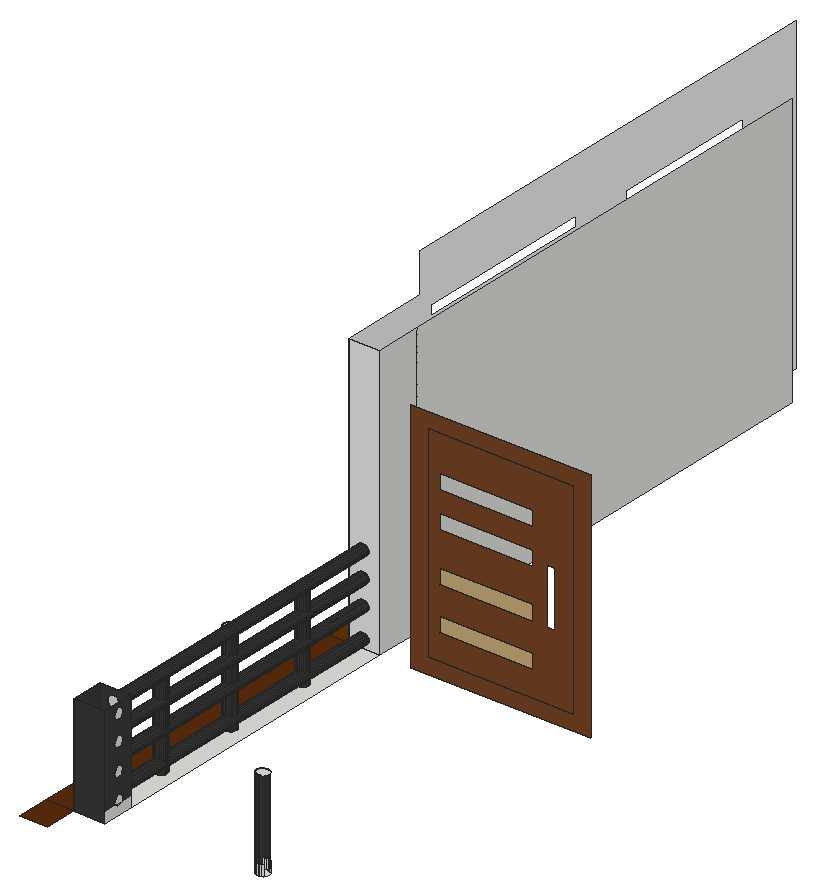
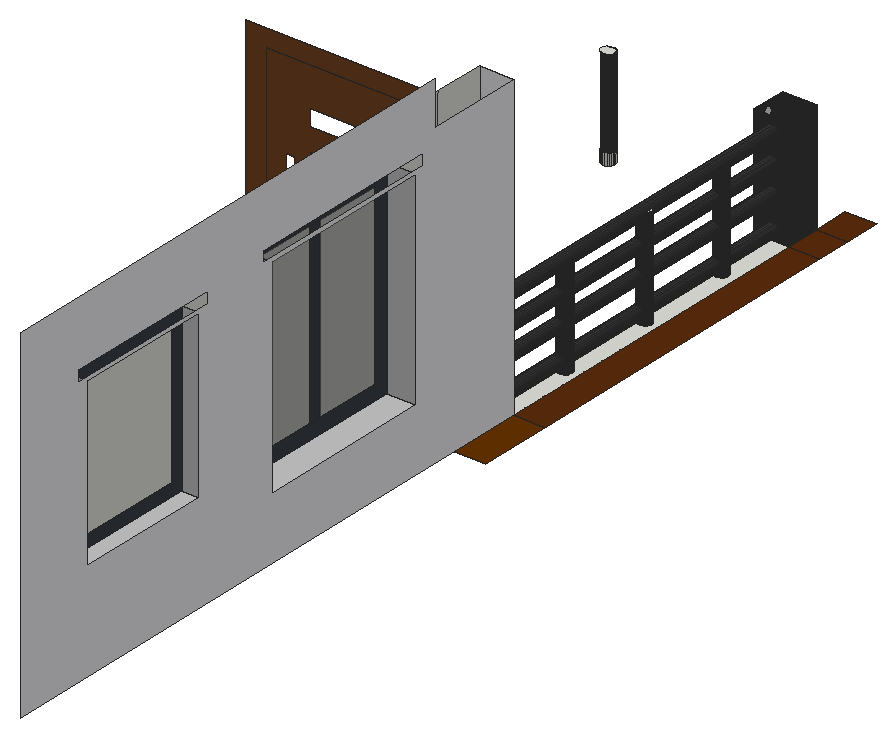
# SketchUp Ruby script. Lengths in inches.
U = 1.inch
M = Sketchup.active_model
def pt(a) = Geom::Point3d.new(a.map { |v| v * U })
def face(e, loops, mat)
  f = e.add_face(loops[0].map { |a| pt(a) })
  loops[1..].each { |l| e.add_face(l.map { |a| pt(a) }).erase! }
  f.material = f.back_material = mat if mat
  f
end
# faces: each face lists its corners as indices into pts; further lists are holes
def faces(e, pts, list, mat = nil) = list.each { |f| face(e, (f[0].is_a?(Array) ? f : [f]).map { |l| l.map { |i| pts[i] } }, mat) }
# xy, xz, yz: faces in a plane at the given z, y or x. An outline is a flat list of corners, or four numbers for a rectangle; further outlines are holes
def ring(l) = l.size == 4 ? [[l[0], l[1]], [l[2], l[1]], [l[2], l[3]], [l[0], l[3]]] : l.each_slice(2).to_a
def flat(e, list, mat, &to3) = list.each { |f| face(e, (f[0].is_a?(Array) ? f : [f]).map { |l| ring(l).map { |u, v| to3.(u, v) } }, mat) }
def xy(e, z, list, mat = nil) = flat(e, list, mat) { |x, y| [x, y, z] }
def xz(e, y, list, mat = nil) = flat(e, list, mat) { |x, z| [x, y, z] }
def yz(e, x, list, mat = nil) = flat(e, list, mat) { |y, z| [x, y, z] }
def lines(e, pts, list) = list.each { |a, b| e.add_line(pt(pts[a]), pt(pts[b])) }
# prism: a flat outline (further loops are holes) pulled along v
def prism(e, loops, v, mat = nil)
  f = face(e, loops, mat); d = Geom::Vector3d.new(v.map { |x| x * U })
  f.pushpull(f.normal.samedirection?(d) ? d.length : -d.length)
end
def box(e, o, s, mat = nil) = prism(e, [[o, [o[0] + s[0], o[1], o[2]], [o[0] + s[0], o[1] + s[1], o[2]], [o[0], o[1] + s[1], o[2]]]], [0, 0, s[2]], mat)
def at(x, y, z, deg = 0) = Geom::Transformation.translation(pt([x, y, z])) * Geom::Transformation.rotation(ORIGIN, Z_AXIS, deg.degrees)
def axes(o, x, y, z) = Geom::Transformation.new([*x, 0, *y, 0, *z, 0, *pt(o).to_a, 1])
def part(name) = M.definitions.add(name)
# library, detail: a bought-in or finely detailed component or shape, given as its bounding box
def library(name, o, s) = part(name).tap { |d| box(d.entities, o, s) }
def detail(e, o, s) = box(e.add_group.entities, o, s)
def put(e, d, t, mat = nil) = e.add_instance(d, t).tap { |i| i.material = mat if mat }
def group(e, t, mat = nil) = e.add_group.tap { |g| g.transformation = t; g.material = mat if mat }.entities
root = M.entities
M.materials.add("[0043_SaddleBrown]").color = [91, 44, 12]
M.materials.add("[Blinds Vertical Pattern]").color = [237, 237, 239]
M.materials.add("[Color C08]").color = [102, 51, 0]
M.materials.add("[Color M02]").color = [198, 198, 198]
M.materials.add("[Color M07]").color = [58, 58, 58]
M.materials.add("[Formica Laminate Dark]").color = [59, 63, 71]
M.materials.add("[Translucent Glass Gray]").color = [128, 128, 128]
M.materials["[Translucent Glass Gray]"].alpha = 0.5
M.materials.add("[Wood Floor Light]").color = [204, 176, 127]
M.materials.add("[Wood Veneer 01]").color = [120, 70, 37]
xy(root,276.4375,[[73.92,405.6875,85.98,418.04],[142,409.67,141.36,409.75,140.77,409.97,140.27,410.32,139.875,410.77,139.63,411.3,139.55,411.86,139.63,412.43,139.875,412.96,140.27,413.41,140.77,413.76,141.36,413.98,142,414.05,142.63,413.98,143.22,413.76,143.73,413.41,144.12,412.96,144.37,412.43,144.45,411.86,144.37,411.3,144.12,410.77,143.73,410.32,143.22,409.97,142.63,409.75],[[73.92,418.04,85.98,538.2],[78.62,507.89,77.99,507.96,77.4,508.18,76.89,508.53,76.5,508.98,76.25,509.51,76.17,510.08,76.25,510.64,76.5,511.17,76.89,511.625,77.4,511.97,77.99,512.19,78.62,512.27,79.25,512.19,79.85,511.97,80.35,511.625,80.74,511.17,80.99,510.64,81.07,510.08,80.99,509.51,80.74,508.98,80.35,508.53,79.85,508.18,79.25,507.96],[78.62,473.02,77.99,473.09,77.4,473.31,76.89,473.66,76.5,474.11,76.25,474.64,76.17,475.2,76.25,475.77,76.5,476.3,76.89,476.75,77.4,477.1,77.99,477.32,78.62,477.39,79.25,477.32,79.85,477.1,80.35,476.75,80.74,476.3,80.99,475.77,81.07,475.2,80.99,474.64,80.74,474.11,80.35,473.66,79.85,473.31,79.25,473.09],[78.97,439.08,78.34,439.15,77.75,439.37,77.24,439.72,76.85,440.17,76.6,440.7,76.52,441.27,76.6,441.83,76.85,442.36,77.24,442.8125,77.75,443.16,78.34,443.38,78.97,443.45,79.6,443.38,80.2,443.16,80.7,442.8125,81.09,442.36,81.34,441.83,81.42,441.27,81.34,440.7,81.09,440.17,80.7,439.72,80.2,439.37,79.6,439.15]],[78.97,439.08,78.34,439.15,77.75,439.37,77.24,439.72,76.85,440.17,76.6,440.7,76.52,441.27,76.6,441.83,76.85,442.36,77.24,442.8125,77.75,443.16,78.34,443.38,78.97,443.45,79.6,443.38,80.2,443.16,80.7,442.8125,81.09,442.36,81.34,441.83,81.42,441.27,81.34,440.7,81.09,440.17,80.7,439.72,80.2,439.37,79.6,439.15],[78.62,473.02,77.99,473.09,77.4,473.31,76.89,473.66,76.5,474.11,76.25,474.64,76.17,475.2,76.25,475.77,76.5,476.3,76.89,476.75,77.4,477.1,77.99,477.32,78.62,477.39,79.25,477.32,79.85,477.1,80.35,476.75,80.74,476.3,80.99,475.77,81.07,475.2,80.99,474.64,80.74,474.11,80.35,473.66,79.85,473.31,79.25,473.09],
  [78.62,507.89,77.99,507.96,77.4,508.18,76.89,508.53,76.5,508.98,76.25,509.51,76.17,510.08,76.25,510.64,76.5,511.17,76.89,511.625,77.4,511.97,77.99,512.19,78.62,512.27,79.25,512.19,79.85,511.97,80.35,511.625,80.74,511.17,80.99,510.64,81.07,510.08,80.99,509.51,80.74,508.98,80.35,508.53,79.85,508.18,79.25,507.96]])
xy(root,276.4375,[[63.07,393.34,73.92,405.6875],[63.07,405.6875,73.92,418.04],[63.07,418.04,73.92,538.2]],"[0043_SaddleBrown]")
xy(root,276.4375,[[63.07,538.2,73.92,564.01]],"[Color C08]")
xy(root,298.41,[[73.92,581.05,84.11,644.17]],"[Color M02]")
xy(root,310.3125,[[78.97,439.08,79.6,439.15,80.2,439.37,80.7,439.72,81.09,440.17,81.34,440.7,81.42,441.27,81.34,441.83,81.09,442.36,80.7,442.8125,80.2,443.16,79.6,443.38,78.97,443.45,78.34,443.38,77.75,443.16,77.24,442.8125,76.85,442.36,76.6,441.83,76.52,441.27,76.6,440.7,76.85,440.17,77.24,439.72,77.75,439.37,78.34,439.15],[78.62,507.89,79.25,507.96,79.85,508.18,80.35,508.53,80.74,508.98,80.99,509.51,81.07,510.08,80.99,510.64,80.74,511.17,80.35,511.625,79.85,511.97,79.25,512.19,78.62,512.27,77.99,512.19,77.4,511.97,76.89,511.625,76.5,511.17,76.25,510.64,76.17,510.08,76.25,509.51,76.5,508.98,76.89,508.53,77.4,508.18,77.99,507.96]])
xy(root,311.09,[[73.92,675.92,79.92,724.73]],"[Color M02]")
xy(root,311.3125,[[142,409.67,142.63,409.75,143.22,409.97,143.73,410.32,144.12,410.77,144.37,411.3,144.45,411.86,144.37,412.43,144.12,412.96,143.73,413.41,143.22,413.76,142.63,413.98,142,414.05,141.36,413.98,140.77,413.76,140.27,413.41,139.875,412.96,139.63,412.43,139.55,411.86,139.63,411.3,139.875,410.77,140.27,410.32,140.77,409.97,141.36,409.75]])
xy(root,311.76,[[78.62,473.02,79.25,473.09,79.85,473.31,80.35,473.66,80.74,474.11,80.99,474.64,81.07,475.2,80.99,475.77,80.74,476.3,80.35,476.75,79.85,477.1,79.25,477.32,78.62,477.39,77.99,477.32,77.43,477.11,77.43,473.29,77.99,473.09],[77.43,473.29,77.43,477.11,77.4,477.1,76.89,476.75,76.5,476.3,76.25,475.77,76.17,475.2,76.25,474.64,76.5,474.11,76.89,473.66,77.4,473.31]])
xz(root,405.6875,[[73.92,276.4375,85.98,315.4375]],"[Color M07]")
xz(root,418.04,[[79.49,277.82,80.11,277.9,80.68,278.11,81.18,278.45,81.55,278.89,81.79,279.4,81.875,279.95,81.79,280.5,81.55,281.01,81.18,281.45,80.68,281.79,80.11,282,79.49,282.07,78.88,282,78.3,281.79,77.81,281.45,77.43,281.01,77.19,280.5,77.11,279.95,77.19,279.4,77.43,278.89,77.81,278.45,78.3,278.11,78.88,277.9],[79.49,289.2,80.11,289.27,80.68,289.48,81.18,289.82,81.55,290.26,81.79,290.77,81.875,291.32,81.79,291.875,81.55,292.39,81.18,292.83,80.68,293.16,80.11,293.375,79.49,293.45,78.88,293.375,78.3,293.16,77.81,292.83,77.43,292.39,77.19,291.875,77.11,291.32,77.19,290.77,77.43,290.26,77.81,289.82,78.3,289.48,78.88,289.27],[79.49,298.82,80.11,298.9,80.68,299.11,81.18,299.45,81.55,299.89,81.79,300.4,81.875,300.95,81.79,301.5,81.55,302.01,81.18,302.45,80.68,302.79,80.11,303,79.49,303.07,78.88,303,78.3,302.79,77.81,302.45,77.43,302.01,77.19,301.5,77.11,300.95,77.19,300.4,77.43,299.89,77.81,299.45,78.3,299.11,78.88,298.9],[79.49,308.57,80.11,308.65,80.68,308.86,81.18,309.2,81.55,309.64,81.79,310.15,81.875,310.7,81.79,311.25,81.55,311.76,81.18,312.2,80.68,312.54,80.11,312.75,79.49,312.82,78.88,312.75,78.3,312.54,77.81,312.2,77.43,311.76,77.19,311.25,77.11,310.7,77.19,310.15,77.43,309.64,77.81,309.2,78.3,308.86,78.88,308.65]])
xz(root,418.04,[[[73.92,276.4375,85.98,315.4375],[79.49,308.57,80.11,308.65,80.68,308.86,81.18,309.2,81.55,309.64,81.79,310.15,81.875,310.7,81.79,311.25,81.55,311.76,81.18,312.2,80.68,312.54,80.11,312.75,79.49,312.82,78.88,312.75,78.3,312.54,77.81,312.2,77.43,311.76,77.19,311.25,77.11,310.7,77.19,310.15,77.43,309.64,77.81,309.2,78.3,308.86,78.88,308.65],[79.49,289.2,80.11,289.27,80.68,289.48,81.18,289.82,81.55,290.26,81.79,290.77,81.875,291.32,81.79,291.875,81.55,292.39,81.18,292.83,80.68,293.16,80.11,293.375,79.49,293.45,78.88,293.375,78.3,293.16,77.81,292.83,77.43,292.39,77.19,291.875,77.11,291.32,77.19,290.77,77.43,290.26,77.81,289.82,78.3,289.48,78.88,289.27],[79.49,298.82,80.11,298.9,80.68,299.11,81.18,299.45,81.55,299.89,81.79,300.4,81.875,300.95,81.79,301.5,81.55,302.01,81.18,302.45,80.68,302.79,80.11,303,79.49,303.07,78.88,303,78.3,302.79,77.81,302.45,77.43,302.01,77.19,301.5,77.11,300.95,77.19,300.4,77.43,299.89,77.81,299.45,78.3,299.11,78.88,298.9],[79.49,277.82,80.11,277.9,80.68,278.11,81.18,278.45,81.55,278.89,81.79,279.4,81.875,279.95,81.79,280.5,81.55,281.01,81.18,281.45,80.68,281.79,80.11,282,79.49,282.07,78.88,282,78.3,281.79,77.81,281.45,77.43,281.01,77.19,280.5,77.11,279.95,77.19,279.4,77.43,278.89,77.81,278.45,78.3,278.11,78.88,277.9]]],"[Color M07]")
xz(root,538.2,[[[73.92,276.4375,85.98,381.625],[79.49,277.82,78.88,277.9,78.3,278.11,77.81,278.45,77.43,278.89,77.19,279.4,77.11,279.95,77.19,280.5,77.43,281.01,77.81,281.45,78.3,281.79,78.88,282,79.49,282.07,80.11,282,80.68,281.79,81.18,281.45,81.55,281.01,81.79,280.5,81.875,279.95,81.79,279.4,81.55,278.89,81.18,278.45,80.68,278.11,80.11,277.9],[79.49,308.57,78.88,308.65,78.3,308.86,77.81,309.2,77.43,309.64,77.19,310.15,77.11,310.7,77.19,311.25,77.43,311.76,77.81,312.2,78.3,312.54,78.88,312.75,79.49,312.82,80.11,312.75,80.68,312.54,81.18,312.2,81.55,311.76,81.79,311.25,81.875,310.7,81.79,310.15,81.55,309.64,81.18,309.2,80.68,308.86,80.11,308.65],[79.49,289.2,78.88,289.27,78.3,289.48,77.81,289.82,77.43,290.26,77.19,290.77,77.11,291.32,77.19,291.875,77.43,292.39,77.81,292.83,78.3,293.16,78.88,293.375,79.49,293.45,80.11,293.375,80.68,293.16,81.18,292.83,81.55,292.39,81.79,291.875,81.875,291.32,81.79,290.77,81.55,290.26,81.18,289.82,80.68,289.48,80.11,289.27],[79.49,298.82,78.88,298.9,78.3,299.11,77.81,299.45,77.43,299.89,77.19,300.4,77.11,300.95,77.19,301.5,77.43,302.01,77.81,302.45,78.3,302.79,78.88,303,79.49,303.07,80.11,303,80.68,302.79,81.18,302.45,81.55,302.01,81.79,301.5,81.875,300.95,81.79,300.4,81.55,299.89,81.18,299.45,80.68,299.11,80.11,298.9]]],"[Blinds Vertical Pattern]")
xz(root,538.2,[[109.29,292.28,145.13,298.15],[109.29,308.96,145.13,314.84]],"[Wood Floor Light]")
xz(root,538.2,[[[98.05,276.4375,167.49,367.3125],[104.875,282.53,160.67,361.22]],[[104.875,282.53,160.67,361.22],[109.29,341.71,145.13,347.59],[109.29,327.9,145.13,333.78],[109.29,308.96,145.13,314.84],[109.29,292.28,145.13,298.15],[150.45,308.77,153.53,330.52]]],"[Wood Veneer 01]")
xz(root,581.05,[[73.92,298.41,84.11,370.85]],"[Color M02]")
xz(root,644.17,[[73.92,298.41,84.11,370.85]],"[Color M02]")
xz(root,675.92,[[73.92,311.09,79.92,369.09]],"[Color M02]")
xz(root,724.73,[[73.92,311.09,79.92,369.09]],"[Color M02]")
yz(root,73.92,[[[538.2,276.4375,538.2,381.625,572.7,381.625,572.7,397.0625,753.91,397.0625,753.91,276.4375],[581.05,298.41,644.17,370.85],[675.92,311.09,724.73,369.09],[578.07,372.15,647.71,376.02],[672.04,370.21,728.61,374.09]]],"[Blinds Vertical Pattern]")
yz(root,73.92,[[405.6875,276.4375,418.04,315.4375]],"[Color M07]")
yz(root,79.92,[[[675.92,311.09,724.73,369.09],[680.38,315.55,720.28,364.63]]],"[Formica Laminate Dark]")
yz(root,84.11,[[[581.05,298.41,644.17,370.85],[586.26,303.62,638.96,365.64]],[610.33,303.62,614.74,365.64]],"[Formica Laminate Dark]")
yz(root,84.11,[[586.26,303.62,610.33,365.64],[614.74,303.62,638.96,365.64]],"[Translucent Glass Gray]")
yz(root,85.98,[[405.6875,276.4375,405.6875,280.5,411,280.5,411.03,280.46,411.4,280.18,411.82,280.01,412.27,279.95,412.72,280.01,413.15,280.18,413.51,280.46,413.54,280.5,418.04,280.5,418.04,276.4375],[538.2,276.4375,556.28,381.625],[556.28,276.4375,737.09,381.625],[412.27,279.95,411.82,280.01,411.4,280.18,411.03,280.46,411,280.5,413.54,280.5,413.51,280.46,413.15,280.18,412.72,280.01],[411,280.5,410.76,280.82,410.58,281.24,410.52,281.7,410.58,282.15,410.76,282.57,411.03,282.93,411.4,283.21,411.82,283.39,412.27,283.45,412.72,283.39,413.15,283.21,413.51,282.93,413.79,282.57,413.96,282.15,414.02,281.7,413.96,281.24,413.79,280.82,413.54,280.5],
  [412.27,289.88,411.82,289.94,411.4,290.12,411.03,290.4,410.76,290.76,410.58,291.18,410.52,291.63,410.58,292.09,410.76,292.51,411.03,292.87,411.4,293.15,411.82,293.33,412.27,293.38,412.72,293.33,413.15,293.15,413.51,292.87,413.79,292.51,413.96,292.09,414.02,291.63,413.96,291.18,413.79,290.76,413.51,290.4,413.15,290.12,412.72,289.94],[412.27,300.26,411.82,300.32,411.4,300.49,411.03,300.77,410.76,301.13,410.58,301.56,410.52,302.01,410.58,302.46,410.76,302.88,411.03,303.25,411.4,303.53,411.82,303.7,412.27,303.76,412.72,303.7,413.15,303.53,413.51,303.25,413.79,302.88,413.96,302.46,414.02,302.01,413.96,301.56,413.79,301.13,413.51,300.77,413.15,300.49,412.72,300.32],[412.27,309.95,411.82,310.01,411.4,310.18,411.03,310.46,410.76,310.82,410.58,311.24,410.52,311.7,410.58,312.15,410.76,312.57,411.03,312.93,411.4,313.21,411.82,313.39,412.27,313.45,412.72,313.39,413.15,313.21,413.51,312.93,413.79,312.57,413.96,312.15,414.02,311.7,413.96,311.24,413.79,310.82,413.51,310.46,413.15,310.18,412.72,310.01]])
yz(root,85.98,[[[405.6875,280.5,411,280.5,410.76,280.82,410.58,281.24,410.52,281.7,410.58,282.15,410.76,282.57,411.03,282.93,411.4,283.21,411.82,283.39,412.27,283.45,412.72,283.39,413.15,283.21,413.51,282.93,413.79,282.57,413.96,282.15,414.02,281.7,413.96,281.24,413.79,280.82,413.54,280.5,418.04,280.5,418.04,315.4375,405.6875,315.4375],[412.27,309.95,411.82,310.01,411.4,310.18,411.03,310.46,410.76,310.82,410.58,311.24,410.52,311.7,410.58,312.15,410.76,312.57,411.03,312.93,411.4,313.21,411.82,313.39,412.27,313.45,412.72,313.39,413.15,313.21,413.51,312.93,413.79,312.57,413.96,312.15,414.02,311.7,413.96,311.24,413.79,310.82,413.51,310.46,413.15,310.18,412.72,310.01],[412.27,289.88,411.82,289.94,411.4,290.12,411.03,290.4,410.76,290.76,410.58,291.18,410.52,291.63,410.58,292.09,410.76,292.51,411.03,292.87,411.4,293.15,411.82,293.33,412.27,293.38,412.72,293.33,413.15,293.15,413.51,292.87,413.79,292.51,413.96,292.09,414.02,291.63,413.96,291.18,413.79,290.76,413.51,290.4,413.15,290.12,412.72,289.94],[412.27,300.26,411.82,300.32,411.4,300.49,411.03,300.77,410.76,301.13,410.58,301.56,410.52,302.01,410.58,302.46,410.76,302.88,411.03,303.25,411.4,303.53,411.82,303.7,412.27,303.76,412.72,303.7,413.15,303.53,413.51,303.25,413.79,302.88,413.96,302.46,414.02,302.01,413.96,301.56,413.79,301.13,413.51,300.77,413.15,300.49,412.72,300.32]]],"[Color M07]")
p = [[140.77,409.97,276.4375],[141.36,409.75,276.4375],[141.36,409.75,280.5],[140.77,409.97,280.5],[142,409.67,276.4375],[142,409.67,280.5],
  [142.63,409.75,276.4375],[142.63,409.75,280.5],[143.22,409.97,276.4375],[143.22,409.97,280.5],[140.27,410.32,276.4375],[140.27,410.32,280.5],
  [143.73,410.32,276.4375],[143.73,410.32,280.5],[139.875,410.77,276.4375],[139.875,410.77,280.5],[139.63,411.3,276.4375],[139.63,411.3,280.5],
  [139.55,411.86,276.4375],[139.55,411.86,280.5],[139.63,412.43,276.4375],[139.63,412.43,280.5],[139.875,412.96,276.4375],[139.875,412.96,280.5],
  [140.27,413.41,276.4375],[140.27,413.41,280.5],[140.77,413.76,276.4375],[140.77,413.76,280.5],[143.73,413.41,276.4375],[143.22,413.76,276.4375],
  [143.22,413.76,280.5],[143.73,413.41,280.5],[141.36,413.98,276.4375],[141.36,413.98,280.5],[142.63,413.98,276.4375],[142.63,413.98,280.5],
  [142,414.05,276.4375],[142,414.05,280.5],[78.34,439.15,276.4375],[78.97,439.08,276.4375],[78.97,439.08,310.3125],[78.34,439.15,310.3125],
  [79.6,439.15,276.4375],[79.6,439.15,310.3125],[77.75,439.37,276.4375],[77.75,439.37,310.3125],[80.2,439.37,276.4375],[80.2,439.37,310.3125],
  [77.24,439.72,276.4375],[77.24,439.72,310.3125],[80.7,439.72,276.4375],[80.7,439.72,310.3125],[76.85,440.17,276.4375],[76.85,440.17,310.3125],
  [81.09,440.17,276.4375],[81.09,440.17,310.3125],[76.6,440.7,276.4375],[76.6,440.7,310.3125],[81.34,440.7,276.4375],[81.34,440.7,310.3125],
  [76.52,441.27,276.4375],[76.52,441.27,310.3125],[81.42,441.27,276.4375],[81.42,441.27,310.3125],[76.6,441.83,276.4375],[76.6,441.83,310.3125],
  [81.34,441.83,276.4375],[81.34,441.83,310.3125],[76.85,442.36,276.4375],[76.85,442.36,310.3125],[81.09,442.36,276.4375],[81.09,442.36,310.3125],
  [77.24,442.8125,276.4375],[77.24,442.8125,310.3125],[80.7,442.8125,276.4375],[80.7,442.8125,310.3125],[77.75,443.16,276.4375],[77.75,443.16,310.3125],
  [80.2,443.16,276.4375],[80.2,443.16,310.3125],[78.34,443.38,276.4375],[78.34,443.38,310.3125],[79.6,443.38,276.4375],[79.6,443.38,310.3125],
  [78.97,443.45,276.4375],[78.97,443.45,310.3125],[77.99,473.09,276.4375],[78.62,473.02,276.4375],[78.62,473.02,311.76],[77.99,473.09,311.76],
  [79.25,473.09,276.4375],[79.25,473.09,311.76],[77.4,473.31,276.4375],[77.43,473.29,311.76],[77.4,473.31,311.76],[79.85,473.31,276.4375],
  [79.85,473.31,311.76],[76.89,473.66,276.4375],[76.89,473.66,311.76],[80.35,473.66,276.4375],[80.35,473.66,311.76],[76.5,474.11,276.4375],
  [76.5,474.11,311.76],[80.74,474.11,276.4375],[80.74,474.11,311.76],[76.25,474.64,276.4375],[76.25,474.64,311.76],[80.99,474.64,276.4375],
  [80.99,474.64,311.76],[76.17,475.2,276.4375],[76.17,475.2,311.76],[81.07,475.2,276.4375],[81.07,475.2,311.76],[76.25,475.77,276.4375],
  [76.25,475.77,311.76],[80.99,475.77,276.4375],[80.99,475.77,311.76],[76.5,476.3,276.4375],[76.5,476.3,311.76],[80.74,476.3,276.4375],
  [80.74,476.3,311.76],[76.89,476.75,276.4375],[76.89,476.75,311.76],[80.35,476.75,276.4375],[80.35,476.75,311.76],[77.4,477.1,276.4375],
  [77.4,477.1,311.76],[79.85,477.1,276.4375],[79.85,477.1,311.76],[77.99,477.32,276.4375],[77.43,477.11,311.76],[77.99,477.32,311.76],
  [79.25,477.32,276.4375],[79.25,477.32,311.76],[78.62,477.39,276.4375],[78.62,477.39,311.76],[77.99,507.96,276.4375],[78.62,507.89,276.4375],
  [78.62,507.89,310.3125],[77.99,507.96,310.3125],[79.25,507.96,276.4375],[79.25,507.96,310.3125],[77.4,508.18,276.4375],[77.4,508.18,310.3125],
  [79.85,508.18,276.4375],[79.85,508.18,310.3125],[76.89,508.53,276.4375],[76.89,508.53,310.3125],[80.35,508.53,276.4375],[80.35,508.53,310.3125],
  [76.5,508.98,276.4375],[76.5,508.98,310.3125],[80.74,508.98,276.4375],[80.74,508.98,310.3125],[76.25,509.51,276.4375],[76.25,509.51,310.3125],
  [80.99,509.51,276.4375],[80.99,509.51,310.3125],[76.17,510.08,276.4375],[76.17,510.08,310.3125],[81.07,510.08,276.4375],[81.07,510.08,310.3125],
  [76.25,510.64,276.4375],[76.25,510.64,310.3125],[80.99,510.64,276.4375],[80.99,510.64,310.3125],[76.5,511.17,276.4375],[76.5,511.17,310.3125],
  [80.74,511.17,276.4375],[80.74,511.17,310.3125],[76.89,511.625,276.4375],[76.89,511.625,310.3125],[80.35,511.625,276.4375],[80.35,511.625,310.3125],
  [77.4,511.97,276.4375],[77.4,511.97,310.3125],[79.85,511.97,276.4375],[79.85,511.97,310.3125],[77.99,512.19,276.4375],[77.99,512.19,310.3125],
  [79.25,512.19,276.4375],[79.25,512.19,310.3125],[78.62,512.27,276.4375],[78.62,512.27,310.3125],[79.49,418.04,277.82],[78.88,418.04,277.9],
  [78.88,538.2,277.9],[79.49,538.2,277.82],[80.11,418.04,277.9],[80.11,538.2,277.9],[78.3,418.04,278.11],[78.3,538.2,278.11],
  [80.68,418.04,278.11],[80.68,538.2,278.11],[77.81,418.04,278.45],[77.81,538.2,278.45],[81.18,418.04,278.45],[81.18,538.2,278.45],
  [77.43,418.04,278.89],[77.43,538.2,278.89],[81.55,418.04,278.89],[81.55,538.2,278.89],[77.19,418.04,279.4],[77.19,538.2,279.4],
  [81.79,418.04,279.4],[81.79,538.2,279.4],[77.11,418.04,279.95],[77.11,538.2,279.95],[81.875,418.04,279.95],[81.875,538.2,279.95],
  [77.19,418.04,280.5],[77.19,538.2,280.5],[81.79,418.04,280.5],[81.79,538.2,280.5],[140.77,409.97,311.3125],[141.36,409.75,311.3125],
  [142,409.67,311.3125],[142.63,409.75,311.3125],[143.22,409.97,311.3125],[140.27,410.32,311.3125],[139.875,410.77,311.3125],[139.63,411.3,311.3125],
  [139.55,411.86,311.3125],[139.63,412.43,311.3125],[139.875,412.96,311.3125],[140.27,413.41,311.3125],[140.77,413.76,311.3125],[141.36,413.98,311.3125],
  [143.22,413.76,311.3125],[142.63,413.98,311.3125],[142,414.05,311.3125],[77.43,418.04,281.01],[77.43,538.2,281.01],[81.55,418.04,281.01],
  [81.55,538.2,281.01],[77.81,418.04,281.45],[77.81,538.2,281.45],[81.18,418.04,281.45],[81.18,538.2,281.45],[78.3,418.04,281.79],
  [78.3,538.2,281.79],[80.68,418.04,281.79],[80.68,538.2,281.79],[78.88,418.04,282],[78.88,538.2,282],[80.11,418.04,282],
  [80.11,538.2,282],[79.49,418.04,282.07],[79.49,538.2,282.07],[79.49,418.04,289.2],[78.88,418.04,289.27],[78.88,538.2,289.27],
  [79.49,538.2,289.2],[80.11,418.04,289.27],[80.11,538.2,289.27],[78.3,418.04,289.48],[78.3,538.2,289.48],[80.68,418.04,289.48],
  [80.68,538.2,289.48],[77.81,418.04,289.82],[77.81,538.2,289.82],[81.18,418.04,289.82],[81.18,538.2,289.82],[77.43,418.04,290.26],
  [77.43,538.2,290.26],[81.55,418.04,290.26],[81.55,538.2,290.26],[77.19,418.04,290.77],[77.19,538.2,290.77],[81.79,418.04,290.77],
  [81.79,538.2,290.77],[77.11,418.04,291.32],[77.11,538.2,291.32],[81.875,418.04,291.32],[81.875,538.2,291.32],[77.19,418.04,291.875],
  [77.19,538.2,291.875],[81.79,418.04,291.875],[81.79,538.2,291.875],[77.43,418.04,292.39],[77.43,538.2,292.39],[81.55,418.04,292.39],
  [81.55,538.2,292.39],[77.81,418.04,292.83],[77.81,538.2,292.83],[81.18,418.04,292.83],[81.18,538.2,292.83],[78.3,418.04,293.16],
  [78.3,538.2,293.16],[80.68,418.04,293.16],[80.68,538.2,293.16],[78.88,418.04,293.375],[78.88,538.2,293.375],[80.11,418.04,293.375],
  [80.11,538.2,293.375],[79.49,418.04,293.45],[79.49,538.2,293.45],[79.49,418.04,298.82],[78.88,418.04,298.9],[78.88,538.2,298.9],
  [79.49,538.2,298.82],[80.11,418.04,298.9],[80.11,538.2,298.9],[78.3,418.04,299.11],[78.3,538.2,299.11],[80.68,418.04,299.11],
  [80.68,538.2,299.11],[77.81,418.04,299.45],[77.81,538.2,299.45],[81.18,418.04,299.45],[81.18,538.2,299.45],[77.43,418.04,299.89],
  [77.43,538.2,299.89],[81.55,418.04,299.89],[81.55,538.2,299.89],[77.19,418.04,300.4],[77.19,538.2,300.4],[81.79,418.04,300.4],
  [81.79,538.2,300.4],[77.11,418.04,300.95],[77.11,538.2,300.95],[81.875,418.04,300.95],[81.875,538.2,300.95],[77.19,418.04,301.5],
  [77.19,538.2,301.5],[81.79,418.04,301.5],[81.79,538.2,301.5],[77.43,418.04,302.01],[77.43,538.2,302.01],[81.55,418.04,302.01],
  [81.55,538.2,302.01],[77.81,418.04,302.45],[77.81,538.2,302.45],[81.18,418.04,302.45],[81.18,538.2,302.45],[78.3,418.04,302.79],
  [78.3,538.2,302.79],[80.68,418.04,302.79],[80.68,538.2,302.79],[78.88,418.04,303],[78.88,538.2,303],[80.11,418.04,303],
  [80.11,538.2,303],[79.49,418.04,303.07],[79.49,538.2,303.07],[78.88,418.04,308.65],[78.3,418.04,308.86],[78.3,538.2,308.86],
  [78.88,538.2,308.65],[79.49,418.04,308.57],[79.49,538.2,308.57],[80.11,418.04,308.65],[80.11,538.2,308.65],[80.68,418.04,308.86],
  [80.68,538.2,308.86],[77.81,418.04,309.2],[77.81,538.2,309.2],[81.18,418.04,309.2],[81.18,538.2,309.2],[77.43,418.04,309.64],
  [77.43,538.2,309.64],[81.55,418.04,309.64],[81.55,538.2,309.64],[77.19,418.04,310.15],[77.19,538.2,310.15],[81.79,418.04,310.15],
  [81.79,538.2,310.15],[77.11,418.04,310.7],[77.11,538.2,310.7],[81.875,418.04,310.7],[81.875,538.2,310.7],[77.19,418.04,311.25],
  [77.19,538.2,311.25],[81.79,418.04,311.25],[81.79,538.2,311.25],[77.43,418.04,311.76],[77.43,538.2,311.76],[81.55,418.04,311.76],
  [81.55,538.2,311.76],[77.81,418.04,312.2],[77.81,538.2,312.2],[81.18,418.04,312.2],[81.18,538.2,312.2],[78.3,418.04,312.54],
  [78.3,538.2,312.54],[80.68,418.04,312.54],[80.68,538.2,312.54],[78.88,418.04,312.75],[78.88,538.2,312.75],[80.11,418.04,312.75],
  [80.11,538.2,312.75],[79.49,418.04,312.82],[79.49,538.2,312.82]]
faces(root,p,[[0,1,2,3],[1,4,5,2],[4,6,7,5],[6,8,9,7],[10,0,3,11],[8,12,13,9],[14,10,11,15],[16,14,15,17],
  [18,16,17,19],[20,18,19,21],[22,20,21,23],[24,22,23,25],[26,24,25,27],[28,29,30,31],[32,26,27,33],[29,34,35,30],
  [36,32,33,37],[34,36,37,35]])
faces(root,p,[[38,39,40,41],[39,42,43,40],[44,38,41,45],[42,46,47,43],[48,44,45,49],[46,50,51,47],[52,48,49,53],[50,54,55,51],
  [56,52,53,57],[54,58,59,55],[60,56,57,61],[58,62,63,59],[64,60,61,65],[62,66,67,63],[68,64,65,69],[66,70,71,67],
  [72,68,69,73],[70,74,75,71],[76,72,73,77],[74,78,79,75],[80,76,77,81],[78,82,83,79],[84,80,81,85],[82,84,85,83],
  [86,87,88,89],[87,90,91,88],[92,86,89,93,94],[90,95,96,91],[97,92,94,98],[95,99,100,96],[101,97,98,102],[99,103,104,100],
  [105,101,102,106],[103,107,108,104],[109,105,106,110],[107,111,112,108],[113,109,110,114],[111,115,116,112],[117,113,114,118],[115,119,120,116],
  [121,117,118,122],[119,123,124,120],[125,121,122,126],[123,127,128,124],[129,125,126,130,131],[127,132,133,128],[134,129,131,135],[132,134,135,133],
  [136,137,138,139],[137,140,141,138],[142,136,139,143],[140,144,145,141],[146,142,143,147],[144,148,149,145],[150,146,147,151],[148,152,153,149],
  [154,150,151,155],[152,156,157,153],[158,154,155,159],[156,160,161,157],[162,158,159,163],[160,164,165,161],[166,162,163,167],[164,168,169,165],
  [170,166,167,171],[168,172,173,169],[174,170,171,175],[172,176,177,173],[178,174,175,179],[176,180,181,177],[182,178,179,183],[180,182,183,181],
  [184,185,186,187],[188,184,187,189],[185,190,191,186],[192,188,189,193],[190,194,195,191],[196,192,193,197],[194,198,199,195],[200,196,197,201],
  [198,202,203,199],[204,200,201,205],[202,206,207,203],[208,204,205,209],[206,210,211,207],[212,208,209,213],[214,3,2,215],[215,2,5,216],
  [216,5,7,217],[217,7,9,218],[219,11,3,214],[220,15,11,219],[221,17,15,220],[222,19,17,221],[223,21,19,222],[224,23,21,223],
  [225,25,23,224],[226,27,25,225],[227,33,27,226],[228,30,35,229],[230,37,33,227],[229,35,37,230],[210,231,232,211],[233,212,213,234],
  [231,235,236,232],[237,233,234,238],[235,239,240,236],[241,237,238,242],[239,243,244,240],[245,241,242,246],[243,247,248,244],[247,245,246,248],
  [249,250,251,252],[253,249,252,254],[250,255,256,251],[257,253,254,258],[255,259,260,256],[261,257,258,262],[259,263,264,260],[265,261,262,266],
  [263,267,268,264],[269,265,266,270],[267,271,272,268],[273,269,270,274],[271,275,276,272],[277,273,274,278],[275,279,280,276],[281,277,278,282],
  [279,283,284,280],[285,281,282,286],[283,287,288,284],[289,285,286,290],[287,291,292,288],[293,289,290,294],[291,295,296,292],[295,293,294,296],
  [297,298,299,300],[301,297,300,302],[298,303,304,299],[305,301,302,306],[303,307,308,304],[309,305,306,310],[307,311,312,308],[313,309,310,314],
  [311,315,316,312],[317,313,314,318],[315,319,320,316],[321,317,318,322],[319,323,324,320],[325,321,322,326],[323,327,328,324],[329,325,326,330],
  [327,331,332,328],[333,329,330,334],[331,335,336,332],[337,333,334,338],[335,339,340,336],[341,337,338,342],[339,343,344,340],[343,341,342,344],
  [345,346,347,348],[349,345,348,350],[351,349,350,352],[353,351,352,354],[346,355,356,347],[357,353,354,358],[355,359,360,356],[361,357,358,362],
  [359,363,364,360],[365,361,362,366],[363,367,368,364],[369,365,366,370],[367,371,372,368],[373,369,370,374],[371,375,93,130,376,372],[377,373,374,378],
  [375,379,380,376,130,93],[381,377,378,382],[379,383,384,380],[385,381,382,386],[383,387,388,384],[389,385,386,390],[387,391,392,388],[391,389,390,392]],"[Color M07]")
